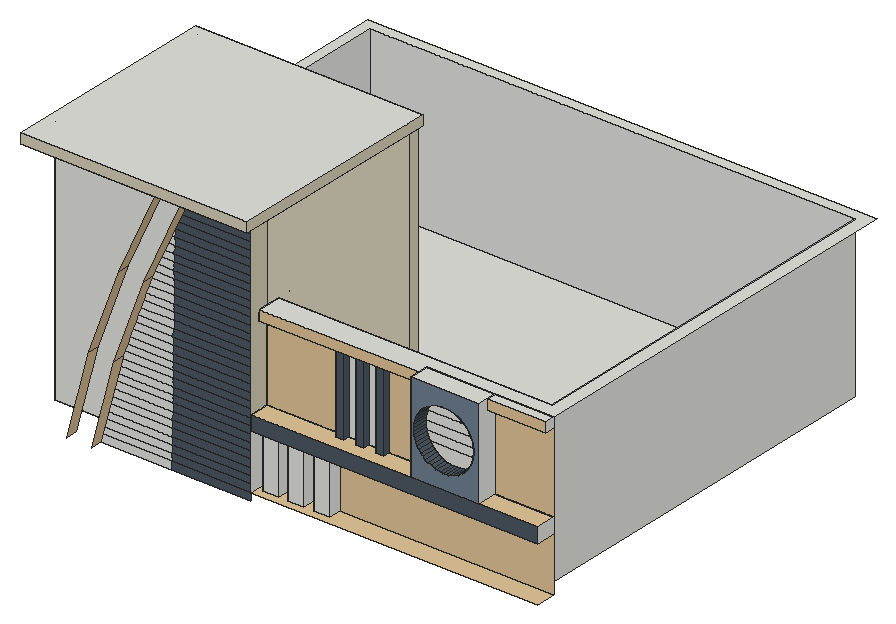
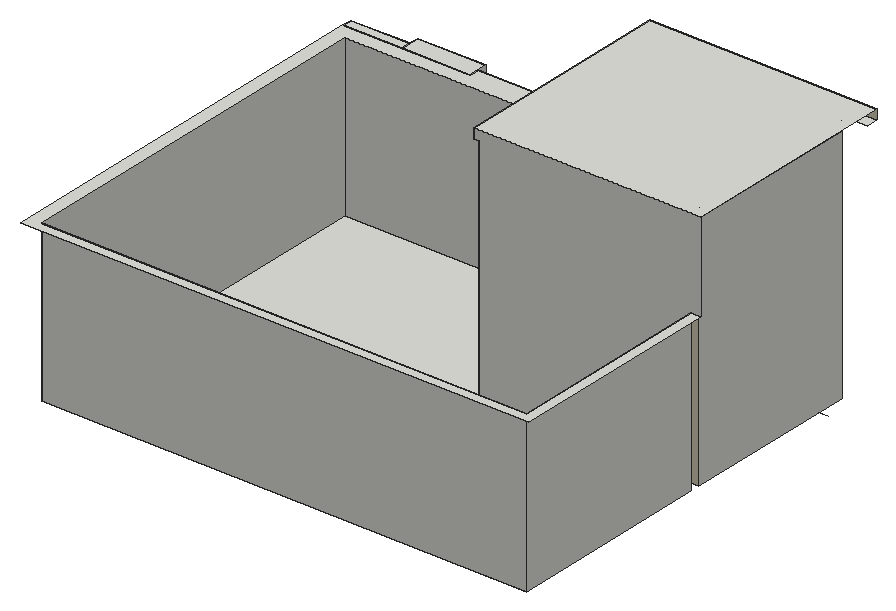
# SketchUp Ruby script. Lengths in inches.
U = 1.inch
M = Sketchup.active_model
def pt(a) = Geom::Point3d.new(a.map { |v| v * U })
def face(e, loops, mat)
  f = e.add_face(loops[0].map { |a| pt(a) })
  loops[1..].each { |l| e.add_face(l.map { |a| pt(a) }).erase! }
  f.material = f.back_material = mat if mat
  f
end
# faces: each face lists its corners as indices into pts; further lists are holes
def faces(e, pts, list, mat = nil) = list.each { |f| face(e, (f[0].is_a?(Array) ? f : [f]).map { |l| l.map { |i| pts[i] } }, mat) }
# xy, xz, yz: faces in a plane at the given z, y or x. An outline is a flat list of corners, or four numbers for a rectangle; further outlines are holes
def ring(l) = l.size == 4 ? [[l[0], l[1]], [l[2], l[1]], [l[2], l[3]], [l[0], l[3]]] : l.each_slice(2).to_a
def flat(e, list, mat, &to3) = list.each { |f| face(e, (f[0].is_a?(Array) ? f : [f]).map { |l| ring(l).map { |u, v| to3.(u, v) } }, mat) }
def xy(e, z, list, mat = nil) = flat(e, list, mat) { |x, y| [x, y, z] }
def xz(e, y, list, mat = nil) = flat(e, list, mat) { |x, z| [x, y, z] }
def yz(e, x, list, mat = nil) = flat(e, list, mat) { |y, z| [x, y, z] }
def lines(e, pts, list) = list.each { |a, b| e.add_line(pt(pts[a]), pt(pts[b])) }
# prism: a flat outline (further loops are holes) pulled along v
def prism(e, loops, v, mat = nil)
  f = face(e, loops, mat); d = Geom::Vector3d.new(v.map { |x| x * U })
  f.pushpull(f.normal.samedirection?(d) ? d.length : -d.length)
end
def box(e, o, s, mat = nil) = prism(e, [[o, [o[0] + s[0], o[1], o[2]], [o[0] + s[0], o[1] + s[1], o[2]], [o[0], o[1] + s[1], o[2]]]], [0, 0, s[2]], mat)
def at(x, y, z, deg = 0) = Geom::Transformation.translation(pt([x, y, z])) * Geom::Transformation.rotation(ORIGIN, Z_AXIS, deg.degrees)
def axes(o, x, y, z) = Geom::Transformation.new([*x, 0, *y, 0, *z, 0, *pt(o).to_a, 1])
def part(name) = M.definitions.add(name)
# library, detail: a bought-in or finely detailed component or shape, given as its bounding box
def library(name, o, s) = part(name).tap { |d| box(d.entities, o, s) }
def detail(e, o, s) = box(e.add_group.entities, o, s)
def put(e, d, t, mat = nil) = e.add_instance(d, t).tap { |i| i.material = mat if mat }
def group(e, t, mat = nil) = e.add_group.tap { |g| g.transformation = t; g.material = mat if mat }.entities
root = M.entities
M.materials.add("[0033_NavajoWhite]").color = [226, 197, 153]
M.materials.add("[0051_Cornsilk]").color = [214, 208, 184]
M.materials.add("[0111_SlateGray]").color = [77, 88, 99]
M.materials.add("[0111_SlateGray]1").color = [112, 128, 144]
xy(root,1740,[[547.78,136.125,586.45,166.125],[24,166.125,534.32,166.125,534.32,201.125,1192.5625,201.125,1192.5625,1114.125,24,1114.125,24,619,534.32,619,534.32,595,24,595]])
xy(root,1740,[[534.32,118.125,1224,118.125,1224,166.125,709.26,166.125,709.26,136.125,670.59,136.125,670.59,166.125,647.2,166.125,647.2,136.125,608.53,136.125,608.53,166.125,586.45,166.125,586.45,136.125,547.78,136.125,547.78,166.125,534.32,166.125]],"[0033_NavajoWhite]")
xy(root,1872,[[547.78,136.125,586.45,166.125],[608.53,136.125,647.2,166.125],[670.59,136.125,709.26,166.125]])
xy(root,1872,[[534.32,118.125,534.32,166.125,547.78,166.125,547.78,136.125,586.45,136.125,586.45,166.125,608.53,166.125,608.53,136.125,647.2,136.125,647.2,166.125,670.59,166.125,670.59,136.125,709.26,136.125,709.26,166.125,1224,166.125,1224,118.125]],"[0033_NavajoWhite]")
xy(root,1908,[[918.28,118.125,1083.04,166.125],[712.94,150.53,730.94,166.125],[761.69,150.53,779.69,166.125],[809.69,150.53,827.69,166.125]])
xy(root,1908,[[534.32,118.125,918.28,118.125,918.28,166.125,827.69,166.125,827.69,150.53,809.69,150.53,809.69,166.125,779.69,166.125,779.69,150.53,761.69,150.53,761.69,166.125,730.94,166.125,730.94,150.53,712.94,150.53,712.94,166.125,534.32,166.125],[1083.04,118.125,1224,166.125]],"[0033_NavajoWhite]")
xy(root,2100,[[712.94,150.53,730.94,166.125],[809.69,150.53,827.69,166.125]])
xy(root,2100,[[534.32,142.125,534.32,166.125,712.94,166.125,712.94,150.53,730.94,150.53,730.94,166.125,761.69,166.125,761.69,150.53,779.69,150.53,779.69,166.125,809.69,166.125,809.69,150.53,827.69,150.53,827.69,166.125,918.28,166.125,918.28,142.125],[1083.04,142.125,1224,166.125]],"[0033_NavajoWhite]")
xy(root,2124,[[918.28,118.125,1083.04,166.125],[534.32,142.125,918.28,142.125,918.28,166.125,1224,166.125,1224,1138.125,0,1138.125,0,619,24,619,24,1114.125,1192.5625,1114.125,1192.5625,201.125,534.32,201.125],[1083.04,142.125,1224,166.125]])
xy(root,2316,[[0,91.125,324,118.125],[384,91.125,534.32,118.125],[534.32,91.125,546.32,166.125],[24,166.125,546.32,595],[534.32,595,546.32,619]])
xy(root,2340,[[0,91.125,546.32,619]])
xz(root,91.125,[[0,2316,546.32,2340]],"[0051_Cornsilk]")
xz(root,118.125,[[171.42,1722,342.85,1722,343.09,1740,176.23,1740],[176.23,1740,343.09,1740,343.33,1758,181.04,1758],[181.04,1758,343.33,1758,343.58,1776,185.85,1776],[185.85,1776,343.58,1776,343.82,1794,190.66,1794],[190.66,1794,343.82,1794,344.0625,1812,195.47,1812],
  [195.47,1812,344.0625,1812,344.31,1830,200.28,1830],[200.28,1830,344.31,1830,344.55,1848,205.09,1848],[205.09,1848,344.55,1848,344.79,1866,209.9,1866],[209.9,1866,344.79,1866,345.03,1884,214.71,1884],[214.71,1884,345.03,1884,345.28,1902,219.52,1902],
  [219.52,1902,345.28,1902,345.52,1920,224.32,1920],[224.32,1920,345.52,1920,345.76,1938,230.28,1938,225.74,1925.31],[230.28,1938,345.76,1938,346.01,1956,236.72,1956],[236.72,1956,346.01,1956,346.25,1974,243.17,1974],[243.17,1974,346.25,1974,346.49,1992,249.61,1992],
  [249.61,1992,346.49,1992,346.74,2010,256.05,2010],[256.05,2010,346.74,2010,346.98,2028,262.49,2028],[262.49,2028,346.98,2028,347.22,2046,268.93,2046],[268.93,2046,347.22,2046,347.47,2064,275.37,2064],[275.37,2064,347.47,2064,347.71,2082,281.81,2082],
  [281.81,2082,347.71,2082,347.95,2100,288.25,2100],[288.25,2100,347.95,2100,348.19,2118,294.6875,2118],[294.6875,2118,348.19,2118,348.4375,2136,302.29,2136,296.81,2123.92],[302.29,2136,348.4375,2136,348.68,2154,310.46,2154],[310.46,2154,348.68,2154,348.92,2172,318.63,2172],
  [318.63,2172,348.92,2172,349.17,2190,326.8,2190],[326.8,2190,349.17,2190,349.41,2208,334.97,2208],[334.97,2208,349.41,2208,349.65,2226,343.14,2226],[343.14,2226,349.65,2226,349.85,2240.77]])
xz(root,118.125,[[342.85,1722,534.32,1722,534.32,1740,343.09,1740],[343.09,1740,534.32,1740,534.32,1758,343.33,1758],[343.33,1758,534.32,1758,534.32,1776,343.58,1776],[343.58,1776,534.32,1776,534.32,1794,343.82,1794],[343.82,1794,534.32,1794,534.32,1812,344.0625,1812],
  [344.0625,1812,534.32,1812,534.32,1830,344.31,1830],[344.31,1830,534.32,1830,534.32,1848,344.55,1848],[344.55,1848,534.32,1848,534.32,1866,344.79,1866],[344.79,1866,534.32,1866,534.32,1884,345.03,1884],[534.32,1872,1224,1908],
  [345.03,1884,534.32,1884,534.32,1902,345.28,1902],[345.28,1902,534.32,1902,534.32,1920,345.52,1920],[345.52,1920,534.32,1920,534.32,1938,345.76,1938],[345.76,1938,534.32,1938,534.32,1956,346.01,1956],[346.01,1956,534.32,1956,534.32,1974,346.25,1974],
  [346.25,1974,534.32,1974,534.32,1992,346.49,1992],[346.49,1992,534.32,1992,534.32,2010,346.74,2010],[346.74,2010,534.32,2010,534.32,2028,346.98,2028],[346.98,2028,534.32,2028,534.32,2046,347.22,2046],[347.22,2046,534.32,2046,534.32,2064,347.47,2064],
  [347.47,2064,534.32,2064,534.32,2082,347.71,2082],[347.71,2082,534.32,2082,534.32,2100,347.95,2100],[347.95,2100,534.32,2100,534.32,2118,348.19,2118],[348.19,2118,534.32,2118,534.32,2136,348.4375,2136],[348.4375,2136,534.32,2136,534.32,2154,348.68,2154],
  [348.68,2154,534.32,2154,534.32,2172,348.92,2172],[348.92,2172,534.32,2172,534.32,2190,349.17,2190],[349.17,2190,534.32,2190,534.32,2208,349.41,2208],[349.41,2208,534.32,2208,534.32,2226,349.65,2226],[349.65,2226,534.32,2226,534.32,2244,351.32,2244,349.85,2240.77],
  [351.32,2244,534.32,2244,534.32,2262,359.49,2262],[359.49,2262,534.32,2262,534.32,2280,367.66,2280],[367.66,2280,534.32,2280,534.32,2298,375.83,2298],[375.83,2298,534.32,2298,534.32,2316,384,2316]],"[0111_SlateGray]")
xz(root,118.125,[[[918.28,1908,1083.04,2124],[995.17,1943.02,987.66,1943.72,980.27,1945.2,973.08,1947.45,966.16,1950.43,959.59,1954.12,953.4375,1958.48,947.78,1963.45,942.67,1968.99,938.17,1975.04,934.32,1981.52,931.17,1988.37,928.76,1995.5,927.11,2002.86,926.23,2010.34,926.14,2017.88,926.84,2025.38,928.32,2032.77,930.5625,2039.97,933.55,2046.89,937.24,2053.46,941.59,2059.61,946.57,2065.27,952.11,2070.38,958.15,2074.88,964.63,2078.72,971.48,2081.87,978.62,2084.29,985.97,2085.9375,993.46,2086.82,1001,2086.91,1008.5,2086.21,1015.89,2084.73,1023.08,2082.48,1030,2079.5,1036.58,2075.81,1042.72,2071.45,1048.38,2066.48,1053.49,2060.9375,1058,2054.89,1061.84,2048.41,1064.99,2041.5625,1067.4,2034.42,1069.06,2027.07,1069.93,2019.59,1070.02,2012.05,1069.32,2004.55,1067.84,1997.16,1065.6,1989.96,1062.62,1983.04,1058.93,1976.47,1054.57,1970.32,1049.59,1964.66,1044.05,1959.55,1038.01,1955.05,1031.53,1951.2,1024.68,1948.06,1017.54,1945.64,1010.1875,1943.99,1002.7,1943.11]]],"[0111_SlateGray]1")
xz(root,136.125,[[547.78,1740,586.45,1872],[608.53,1740,647.2,1872],[670.59,1740,709.26,1872]])
xz(root,142.125,[[534.32,2100,918.28,2124],[1083.04,2100,1224,2124]],"[0033_NavajoWhite]")
xz(root,150.53,[[712.94,1908,730.94,2100],[761.69,1908,779.69,2100],[809.69,1908,827.69,2100]],"[0111_SlateGray]")
xz(root,154.125,[[995.17,1943.02,1002.7,1943.11,1010.1875,1943.99,1017.54,1945.64,1024.68,1948.06,1031.53,1951.2,1038.01,1955.05,1044.05,1959.55,1049.59,1964.66,1054.57,1970.32,1058.93,1976.47,937.32,1976.47,938.17,1975.04,942.67,1968.99,947.78,1963.45,953.4375,1958.48,959.59,1954.12,966.16,1950.43,973.08,1947.45,980.27,1945.2,987.66,1943.72],[937.32,1976.47,1058.93,1976.47,1062.62,1983.04,1065.6,1989.96,1067.84,1997.16,928.39,1997.16,928.76,1995.5,931.17,1988.37,934.32,1981.52],[928.39,1997.16,1067.84,1997.16,1069.32,2004.55,1070.02,2012.05,1069.93,2019.59,926.3,2019.59,926.14,2017.88,926.23,2010.34,927.11,2002.86],[926.3,2019.59,1069.93,2019.59,1069.06,2027.07,1067.4,2034.42,1065.04,2041.41,931.18,2041.41,930.5625,2039.97,928.32,2032.77,926.84,2025.38],[931.18,2041.41,1065.04,2041.41,1064.99,2041.5625,1061.84,2048.41,1058,2054.89,1053.49,2060.9375,1048.38,2066.48,947.88,2066.48,946.57,2065.27,941.59,2059.61,937.24,2053.46,934.4,2048.41,933.55,2046.89],
  [947.88,2066.48,1048.38,2066.48,1042.72,2071.45,1036.58,2075.81,1030,2079.5,1023.08,2082.48,1015.89,2084.73,1008.5,2086.21,1001,2086.91,993.46,2086.82,985.97,2085.9375,978.62,2084.29,971.48,2081.87,964.63,2078.72,958.15,2074.88,952.11,2070.38]])
xz(root,166.125,[[24,1740,24,2316,534.32,2316,534.32,2124,533.82,2124,533.82,1740],[533.82,1740,534.32,2124],[534.32,1740,547.78,1872],[547.78,1740,586.45,1872],[586.45,1740,608.53,1872],
  [647.2,1740,670.59,1872],[534.32,1872,1224,1908],[712.94,1908,730.94,2100],[730.94,1908,761.69,2100],[779.69,1908,809.69,2100],
  [809.69,1908,827.69,2100],[918.28,1908,1083.04,2124],[1083.04,2100,1224,2124]])
xz(root,166.125,[[709.26,1740,1224,1872],[534.32,1908,712.94,2100],[827.69,1908,918.28,2100],[1083.04,1908,1224,2100]],"[0033_NavajoWhite]")
xz(root,201.125,[[534.32,1740,1192.5625,2124]])
xz(root,595,[[24,1740,534.32,2316]],"[0051_Cornsilk]")
xz(root,619,[[24,1740,24,2124,0,2124,0,2340,546.32,2340,546.32,2316,534.32,2316,534.32,1740]])
xz(root,1114.125,[[24,1740,1192.5625,2124]])
yz(root,24,[[166.125,1740,595,2316],[619,1740,1114.125,2124]])
yz(root,534.32,[[118.125,1740,166.125,1872],[166.125,1740,201.125,2124],[118.125,1872,166.125,1908],[142.125,2100,166.125,2124]])
yz(root,534.32,[[595,1740,619,2316],[118.125,1908,166.125,1908,166.125,2100,142.125,2100,142.125,2124,166.125,2124,166.125,2316,118.125,2316]],"[0051_Cornsilk]")
yz(root,546.32,[[91.125,2316,619,2340]],"[0051_Cornsilk]")
yz(root,547.78,[[136.125,1740,166.125,1872]])
yz(root,586.45,[[136.125,1740,166.125,1872]])
yz(root,608.53,[[136.125,1740,166.125,1872]])
yz(root,647.2,[[136.125,1740,166.125,1872]])
yz(root,670.59,[[136.125,1740,166.125,1872]])
yz(root,709.26,[[136.125,1740,166.125,1872]])
yz(root,712.94,[[150.53,1908,166.125,2100]],"[0111_SlateGray]")
yz(root,730.94,[[150.53,1908,166.125,2100]],"[0111_SlateGray]")
yz(root,761.69,[[150.53,1908,166.125,2100]],"[0111_SlateGray]")
yz(root,779.69,[[150.53,1908,166.125,2100]],"[0111_SlateGray]")
yz(root,809.69,[[150.53,1908,166.125,2100]],"[0111_SlateGray]")
yz(root,827.69,[[150.53,1908,166.125,2100]],"[0111_SlateGray]")
yz(root,918.28,[[118.125,1908,118.125,2124,142.125,2124,142.125,2100,166.125,2100,166.125,1908],[142.125,2100,166.125,2124]])
yz(root,1083.04,[[118.125,1908,166.125,1908,166.125,2100,142.125,2100,142.125,2124,118.125,2124],[142.125,2100,166.125,2124]])
yz(root,1192.5625,[[201.125,1740,1114.125,2124]])
yz(root,1224,[[118.125,1872,166.125,1908],[142.125,2100,166.125,2124]])
p = [[165.74,118.125,1925.31],[111.29,118.125,1721.51],[111.29,91.125,1721.51],[165.74,91.125,1925.31],[224.32,118.125,1920],[225.74,118.125,1925.31],
  [225.74,91.125,1925.31],[171.29,91.125,1721.51],[171.29,118.125,1721.51],[171.42,118.125,1722],[176.23,118.125,1740],[181.04,118.125,1758],
  [185.85,118.125,1776],[190.66,118.125,1794],[195.47,118.125,1812],[200.28,118.125,1830],[205.09,118.125,1848],[209.9,118.125,1866],
  [214.71,118.125,1884],[219.52,118.125,1902],[236.81,118.125,2123.92],[236.81,91.125,2123.92],[294.6875,118.125,2118],[296.81,118.125,2123.92],
  [296.81,91.125,2123.92],[230.28,118.125,1938],[236.72,118.125,1956],[243.17,118.125,1974],[249.61,118.125,1992],[256.05,118.125,2010],
  [262.49,118.125,2028],[268.93,118.125,2046],[275.37,118.125,2064],[281.81,118.125,2082],[288.25,118.125,2100],[987.66,118.125,1943.72],
  [995.17,118.125,1943.02],[995.17,154.125,1943.02],[987.66,154.125,1943.72],[1002.7,118.125,1943.11],[1002.7,154.125,1943.11],[1010.1875,118.125,1943.99],
  [1010.1875,154.125,1943.99],[980.27,118.125,1945.2],[980.27,154.125,1945.2],[1017.54,118.125,1945.64],[1017.54,154.125,1945.64],[973.08,118.125,1947.45],
  [973.08,154.125,1947.45],[1024.68,118.125,1948.06],[1024.68,154.125,1948.06],[966.16,118.125,1950.43],[966.16,154.125,1950.43],[1031.53,118.125,1951.2],
  [1031.53,154.125,1951.2],[959.59,118.125,1954.12],[959.59,154.125,1954.12],[1038.01,118.125,1955.05],[1038.01,154.125,1955.05],[953.4375,118.125,1958.48],
  [953.4375,154.125,1958.48],[1044.05,118.125,1959.55],[1044.05,154.125,1959.55],[947.78,118.125,1963.45],[947.78,154.125,1963.45],[1049.59,118.125,1964.66],
  [1049.59,154.125,1964.66],[942.67,118.125,1968.99],[942.67,154.125,1968.99],[1054.57,118.125,1970.32],[1054.57,154.125,1970.32],[938.17,118.125,1975.04],
  [938.17,154.125,1975.04],[1058.93,118.125,1976.47],[1058.93,154.125,1976.47],[934.32,118.125,1981.52],[937.32,154.125,1976.47],[934.32,154.125,1981.52],
  [1062.62,118.125,1983.04],[1062.62,154.125,1983.04],[931.17,118.125,1988.37],[931.17,154.125,1988.37],[1065.6,118.125,1989.96],[1065.6,154.125,1989.96],
  [928.76,118.125,1995.5],[928.76,154.125,1995.5],[1067.84,118.125,1997.16],[1067.84,154.125,1997.16],[927.11,118.125,2002.86],[928.39,154.125,1997.16],
  [927.11,154.125,2002.86],[1069.32,118.125,2004.55],[1069.32,154.125,2004.55],[926.23,118.125,2010.34],[926.23,154.125,2010.34],[1070.02,118.125,2012.05],
  [1070.02,154.125,2012.05],[926.14,118.125,2017.88],[926.14,154.125,2017.88],[1069.93,118.125,2019.59],[1069.93,154.125,2019.59],[926.84,118.125,2025.38],
  [926.3,154.125,2019.59],[926.84,154.125,2025.38],[1069.06,118.125,2027.07],[1069.06,154.125,2027.07],[928.32,118.125,2032.77],[928.32,154.125,2032.77],
  [1067.4,118.125,2034.42],[1067.4,154.125,2034.42],[930.5625,118.125,2039.97],[930.5625,154.125,2039.97],[1064.99,118.125,2041.5625],[1064.99,154.125,2041.5625],
  [1065.04,154.125,2041.41],[933.55,118.125,2046.89],[931.18,154.125,2041.41],[933.55,154.125,2046.89],[1061.84,118.125,2048.41],[1061.84,154.125,2048.41],
  [937.24,118.125,2053.46],[934.4,154.125,2048.41],[937.24,154.125,2053.46],[1058,118.125,2054.89],[1058,154.125,2054.89],[941.59,118.125,2059.61],
  [941.59,154.125,2059.61],[1053.49,118.125,2060.9375],[1053.49,154.125,2060.9375],[946.57,118.125,2065.27],[946.57,154.125,2065.27],[1048.38,118.125,2066.48],
  [1048.38,154.125,2066.48],[952.11,118.125,2070.38],[947.88,154.125,2066.48],[952.11,154.125,2070.38],[1042.72,118.125,2071.45],[1042.72,154.125,2071.45],
  [958.15,118.125,2074.88],[958.15,154.125,2074.88],[1036.58,118.125,2075.81],[1036.58,154.125,2075.81],[964.63,118.125,2078.72],[964.63,154.125,2078.72],
  [1030,118.125,2079.5],[1030,154.125,2079.5],[971.48,118.125,2081.87],[971.48,154.125,2081.87],[1023.08,118.125,2082.48],[1023.08,154.125,2082.48],
  [978.62,118.125,2084.29],[978.62,154.125,2084.29],[1015.89,118.125,2084.73],[1015.89,154.125,2084.73],[985.97,118.125,2085.9375],[985.97,154.125,2085.9375],
  [1008.5,118.125,2086.21],[1008.5,154.125,2086.21],[993.46,118.125,2086.82],[993.46,154.125,2086.82],[1001,118.125,2086.91],[1001,154.125,2086.91],
  [324,118.125,2316],[324,91.125,2316],[375.83,118.125,2298],[384,118.125,2316],[384,91.125,2316],[302.29,118.125,2136],
  [310.46,118.125,2154],[318.63,118.125,2172],[326.8,118.125,2190],[334.97,118.125,2208],[343.14,118.125,2226],[349.85,118.125,2240.77],
  [351.32,118.125,2244],[359.49,118.125,2262],[367.66,118.125,2280],[24,234.25,1740],[0,234.25,1740],[534.32,234.25,2124],
  [533.82,234.25,2124],[24,166.125,2316],[24,166.125,2340],[24,595,2316],[24,595,2340]]
faces(root,p,[[0,1,2,3],[4,5,6,7,8,9,10,11,12,13,14,15,16,17,18,19],[20,0,3,21],[22,23,24,6,5,25,26,27,28,29,30,31,32,33,34],[162,20,21,163],[164,165,166,24,23,167,168,169,170,171,172,173,174,175,176]],"[0033_NavajoWhite]")
faces(root,p,[[35,36,37,38],[36,39,40,37],[39,41,42,40],[43,35,38,44],[41,45,46,42],[47,43,44,48],[45,49,50,46],[51,47,48,52],
  [49,53,54,50],[55,51,52,56],[53,57,58,54],[59,55,56,60],[57,61,62,58],[63,59,60,64],[61,65,66,62],[67,63,64,68],
  [65,69,70,66],[71,67,68,72],[69,73,74,70],[75,71,72,76,77],[73,78,79,74],[80,75,77,81],[78,82,83,79],[84,80,81,85],
  [82,86,87,83],[88,84,85,89,90],[86,91,92,87],[93,88,90,94],[91,95,96,92],[97,93,94,98],[95,99,100,96],[101,97,98,102,103],
  [99,104,105,100],[106,101,103,107],[104,108,109,105],[110,106,107,111],[108,112,113,114,109],[115,110,111,116,117],[112,118,119,113],[120,115,117,121,122],
  [118,123,124,119],[125,120,122,126],[123,127,128,124],[129,125,126,130],[127,131,132,128],[133,129,130,134,135],[131,136,137,132],[138,133,135,139],
  [136,140,141,137],[142,138,139,143],[140,144,145,141],[146,142,143,147],[144,148,149,145],[150,146,147,151],[148,152,153,149],[154,150,151,155],
  [152,156,157,153],[158,154,155,159],[156,160,161,157],[160,158,159,161]],"[0111_SlateGray]")
lines(root,p,[[177,178],[179,180],[181,182],[183,184]])
